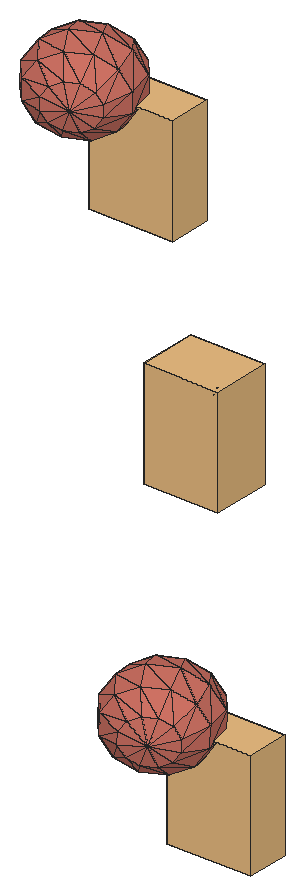
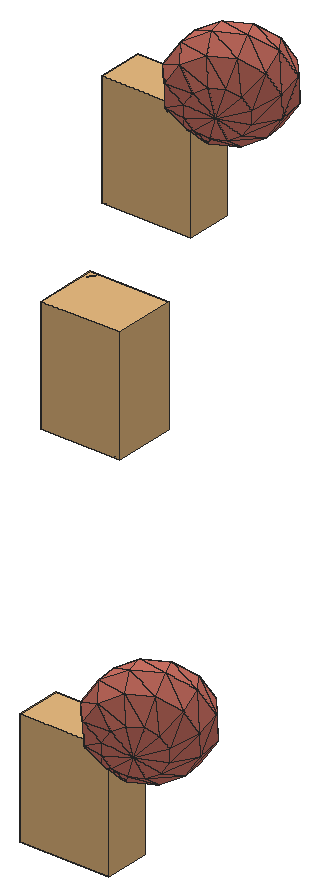
# SketchUp Ruby script. Lengths in inches.
U = 1.inch
M = Sketchup.active_model
def pt(a) = Geom::Point3d.new(a.map { |v| v * U })
def face(e, loops, mat)
  f = e.add_face(loops[0].map { |a| pt(a) })
  loops[1..].each { |l| e.add_face(l.map { |a| pt(a) }).erase! }
  f.material = f.back_material = mat if mat
  f
end
# faces: each face lists its corners as indices into pts; further lists are holes
def faces(e, pts, list, mat = nil) = list.each { |f| face(e, (f[0].is_a?(Array) ? f : [f]).map { |l| l.map { |i| pts[i] } }, mat) }
# xy, xz, yz: faces in a plane at the given z, y or x. An outline is a flat list of corners, or four numbers for a rectangle; further outlines are holes
def ring(l) = l.size == 4 ? [[l[0], l[1]], [l[2], l[1]], [l[2], l[3]], [l[0], l[3]]] : l.each_slice(2).to_a
def flat(e, list, mat, &to3) = list.each { |f| face(e, (f[0].is_a?(Array) ? f : [f]).map { |l| ring(l).map { |u, v| to3.(u, v) } }, mat) }
def xy(e, z, list, mat = nil) = flat(e, list, mat) { |x, y| [x, y, z] }
def xz(e, y, list, mat = nil) = flat(e, list, mat) { |x, z| [x, y, z] }
def yz(e, x, list, mat = nil) = flat(e, list, mat) { |y, z| [x, y, z] }
def lines(e, pts, list) = list.each { |a, b| e.add_line(pt(pts[a]), pt(pts[b])) }
# prism: a flat outline (further loops are holes) pulled along v
def prism(e, loops, v, mat = nil)
  f = face(e, loops, mat); d = Geom::Vector3d.new(v.map { |x| x * U })
  f.pushpull(f.normal.samedirection?(d) ? d.length : -d.length)
end
def box(e, o, s, mat = nil) = prism(e, [[o, [o[0] + s[0], o[1], o[2]], [o[0] + s[0], o[1] + s[1], o[2]], [o[0], o[1] + s[1], o[2]]]], [0, 0, s[2]], mat)
def at(x, y, z, deg = 0) = Geom::Transformation.translation(pt([x, y, z])) * Geom::Transformation.rotation(ORIGIN, Z_AXIS, deg.degrees)
def axes(o, x, y, z) = Geom::Transformation.new([*x, 0, *y, 0, *z, 0, *pt(o).to_a, 1])
def part(name) = M.definitions.add(name)
# library, detail: a bought-in or finely detailed component or shape, given as its bounding box
def library(name, o, s) = part(name).tap { |d| box(d.entities, o, s) }
def detail(e, o, s) = box(e.add_group.entities, o, s)
def put(e, d, t, mat = nil) = e.add_instance(d, t).tap { |i| i.material = mat if mat }
def group(e, t, mat = nil) = e.add_group.tap { |g| g.transformation = t; g.material = mat if mat }.entities
root = M.entities
M.materials.add("green").color = [174, 139, 102]
M.materials.add("vio").color = [206, 114, 100]
c1 = part("3DGeom~219_Defintion")
p = [[167.16,-297.35,-320.32],[-80.93,-262.73,-388.47],[-36.76,-95.49,-489.125],[218.17,-104.25,-436.54],[-281.83,-61.15,-410.64],[-43.21,95.93,-488.48],
  [-285.56,49.37,-410.27],[210.71,116.79,-435.8],[-317.52,144.24,-351.51],[-98.5625,260.26,-386.7],[-98.5625,260.26,-386.7],[370.46,-252.3,-166.34],
  [370.46,-252.3,-166.34],[414.63,-85.07,-266.99],[414.63,-85.07,-266.99],[414.63,-85.07,-266.99],[408.18,106.36,-266.34],[408.18,106.36,-266.34],
  [146.8,306.54,-318.28],[-98.5625,260.26,-386.7],[146.8,306.54,-318.28],[-307.34,-157.7,-352.53],[-281.83,-61.15,-410.64],[-307.34,-157.7,-352.53],
  [-451.39,-10.42,-222.13],[-285.56,49.37,-410.27],[-281.83,-61.15,-410.64],[-317.52,144.24,-351.51],[-285.56,49.37,-410.27],[71.36,-410.78,-118.27],
  [-163.89,-360.96,-213.49],[-80.93,-262.73,-388.47],[-80.93,-262.73,-388.47],[167.16,-297.35,-320.32],[-163.89,-360.96,-213.49],[-98.5625,260.26,-386.7],
  [-369.14,198.04,-250.11],[-98.5625,260.26,-386.7],[-369.14,198.04,-250.11],[-187.98,353.45,-211.07],[146.8,306.54,-318.28],[-98.5625,260.26,-386.7],
  [-187.98,353.45,-211.07],[-163.89,-360.96,-213.49],[-355.23,-214.42,-251.51],[-307.34,-157.7,-352.53],[-355.23,-214.42,-251.51],[-369.14,198.04,-250.11],
  [-317.52,144.24,-351.51],[287.5,-350.53,8.64],[167.16,-297.35,-320.32],[287.5,-350.53,8.64],[167.16,-297.35,-320.32],[370.46,-252.3,-166.34],
  [408.18,106.36,-266.34],[146.8,306.54,-318.28],[352.83,270.68,-164.57],[352.83,270.68,-164.57],[43.55,414.14,-115.47],[474.5,-139.65,32.21],
  [370.46,-252.3,-166.34],[414.63,-85.07,-266.99],[500,-43.09,-25.9],[408.18,106.36,-266.34],[496.27,67.43,-25.53],[352.83,270.68,-164.57],
  [-263.41,-363.87,-11.0625],[-412.69,-216.1,-134.63],[-355.23,-214.42,-251.51],[-355.23,-214.42,-251.51],[-355.23,-214.42,-251.51],[-412.69,-216.1,-134.63],
  [-426.6,196.36,-133.24],[-187.98,353.45,-211.07],[-412.69,-216.1,-134.63],[-464.32,-162.3,-33.23],[-496.27,-67.42,25.53],[-500,43.09,25.9],
  [-474.5,139.65,-32.21],[-43.55,-414.14,115.47],[-187.98,353.45,-211.07],[-287.5,350.54,-8.64],[-287.5,350.54,-8.64],[426.6,-196.36,133.24],
  [287.5,-350.53,8.64],[464.32,162.3,33.23],[263.41,363.87,11.0625],[352.83,270.68,-164.57],[263.41,363.87,11.0625],[-352.83,-270.68,164.57],
  [-412.69,-216.1,-134.63],[-263.41,-363.87,-11.0625],[-352.83,-270.68,164.57],[-412.69,-216.1,-134.63],[-287.5,350.54,-8.64],[187.98,-353.45,211.07],
  [187.98,-353.45,211.07],[287.5,-350.53,8.64],[-71.36,410.78,118.27],[-408.18,-106.36,266.34],[-352.83,-270.68,164.57],[-408.18,-106.36,266.34],
  [-370.46,252.3,166.34],[-287.5,350.54,-8.64],[-370.46,252.3,166.34],[451.39,10.42,222.13],[-146.8,-306.54,318.28],[-146.8,-306.54,318.28],
  [-352.83,-270.68,164.57],[-370.46,252.3,166.34],[369.14,-198.04,250.11],[187.98,-353.45,211.07],[263.41,363.87,11.0625],[412.69,216.1,134.63],
  [412.69,216.1,134.63],[163.89,360.96,213.49],[163.89,360.96,213.49],[-414.63,85.07,266.99],[-408.18,-106.36,266.34],[-414.63,85.07,266.99],
  [-370.46,252.3,166.34],[-414.63,85.07,266.99],[98.5625,-260.26,386.7],[-146.8,-306.54,318.28],[98.5625,-260.26,386.7],[187.98,-353.45,211.07],
  [-370.46,252.3,166.34],[-167.16,297.35,320.32],[163.89,360.96,213.49],[-167.16,297.35,320.32],[355.23,214.42,251.51],[412.69,216.1,134.63],
  [163.89,360.96,213.49],[355.23,214.42,251.51],[-210.71,-116.79,435.8],[-352.83,-270.68,164.57],[-146.8,-306.54,318.28],[-408.18,-106.36,266.34],
  [-167.16,297.35,320.32],[-370.46,252.3,166.34],[-414.63,85.07,266.99],[317.52,-144.24,351.51],[98.5625,-260.26,386.7],[187.98,-353.45,211.07],
  [317.52,-144.24,351.51],[187.98,-353.45,211.07],[369.14,-198.04,250.11],[355.23,214.42,251.51],[163.89,360.96,213.49],[80.93,262.73,388.47],
  [163.89,360.96,213.49],[-167.16,297.35,320.32],[80.93,262.73,388.47],[317.52,-144.24,351.51],[285.56,-49.37,410.27],[281.83,61.15,410.64],
  [307.34,157.7,352.53],[355.23,214.42,251.51],[307.34,157.7,352.53],[-218.17,104.25,436.54],[43.21,-95.93,488.48],[285.56,-49.37,410.27],
  [317.52,-144.24,351.51],[307.34,157.7,352.53],[36.76,95.49,489.125],[281.83,61.15,410.64],[307.34,157.7,352.53],[285.56,-49.37,410.27],
  [281.83,61.15,410.64],[285.56,-49.37,410.27],[281.83,61.15,410.64]]
faces(c1.entities,p,[[0,1,2],[0,2,3],[1,4,2],[3,2,5],[2,4,6],[2,6,5],[3,5,7],[5,6,8],
  [5,8,9],[7,5,10],[11,0,3],[12,3,13],[14,3,7],[15,7,16],[17,7,18],[7,19,20],
  [1,21,4],[22,23,24],[25,26,24],[27,28,24],[29,30,31],[29,32,33],[34,21,1],[35,8,36],
  [37,38,39],[40,41,42],[43,44,21],[45,46,24],[47,48,24],[49,29,50],[51,52,53],[54,55,56],
  [57,40,58],[40,42,58],[59,60,61],[59,61,62],[62,61,63],[62,63,64],[64,63,65],[66,67,68],
  [66,69,30],[70,71,24],[72,47,24],[73,47,72],[74,75,24],[75,76,24],[76,77,24],[77,78,24],
  [78,72,24],[79,66,30],[79,30,29],[80,72,81],[58,42,82],[83,84,60],[83,60,59],[64,65,85],
  [85,65,86],[87,58,88],[89,90,91],[92,75,93],[94,72,78],[95,79,29],[96,29,97],[58,82,98],
  [88,58,98],[99,75,100],[101,76,75],[102,78,77],[103,78,104],[59,62,105],[62,64,105],[64,85,105],
  [106,66,79],[107,108,66],[98,82,109],[110,111,84],[110,84,83],[85,112,113],[114,88,115],[88,98,116],
  [117,76,118],[119,77,76],[120,77,121],[83,59,105],[85,113,105],[122,123,79],[124,79,125],[98,126,127],
  [128,98,129],[110,83,105],[113,130,105],[131,132,133],[134,135,136],[134,137,135],[138,139,140],[141,142,143],
  [144,145,146],[147,148,149],[150,151,152],[153,110,105],[154,153,105],[155,154,105],[156,155,105],[130,156,105],
  [157,149,158],[159,137,134],[159,140,137],[138,140,159],[160,134,136],[160,136,142],[149,138,159],[161,142,162],
  [163,164,165],[166,149,164],[167,160,142],[149,159,164],[168,160,169],[170,164,160],[164,159,134],[164,134,160]],"vio")
c2 = library("3DGeom~96_Defintion",[-195.05,-500,-388.01],[390.1,1000,776.02])
c3 = part("3DGeom~97_Defintion")
p = [[174.48,487.39,-384.2],[155.8125,487.85,-388.01],[137.83,489.88,-382.14],[174.48,487.39,-384.2],[125.36,492.93,-368.18],[121.74,496.1875,-349.85],
  [174.48,487.39,-384.2],[121.74,496.1875,-349.85],[127.94,498.77,-332.09],[174.48,487.39,-384.2],[137.83,489.88,-382.14],[125.36,492.93,-368.18],
  [174.48,487.39,-384.2],[127.94,498.77,-332.09],[142.3,500,-319.63],[174.48,487.39,-384.2],[142.3,500,-319.63],[160.98,499.54,-315.83],
  [174.48,487.39,-384.2],[160.98,499.54,-315.83],[178.96,497.51,-321.7],[174.48,487.39,-384.2],[191.43,494.46,-335.66],[195.05,491.2,-353.98],
  [174.48,487.39,-384.2],[195.05,491.2,-353.98],[188.85,488.61,-371.75],[174.48,487.39,-384.2],[178.96,497.51,-321.7],[191.43,494.46,-335.66],
  [-147.29,-500,333.96],[-182.28,-490.37,332.19],[-165.51,-497.625,329.13],[-182.28,-490.37,332.19],[-147.29,-500,333.96],[-195.05,-469.79,356.79],
  [-182.28,-490.37,332.19],[-195.05,-469.79,356.79],[-193.09,-480.18,342.3125],[-195.05,-469.79,356.79],[-147.29,-500,333.96],[-172.82,-458.84,383.18],
  [-172.82,-458.84,383.18],[-147.29,-500,333.96],[-137.83,-468.47,384.95],[-147.29,-500,333.96],[-132.48,-496.86,345.39],[-125.0625,-489.05,360.34],
  [-137.83,-468.47,384.95],[-147.29,-500,333.96],[-125.0625,-489.05,360.34],[-195.05,-469.79,356.79],[-172.82,-458.84,383.18],[-187.63,-461.98,371.75],
  [-137.83,-468.47,384.95],[-125.0625,-489.05,360.34],[-127.02,-478.66,374.83],[-172.82,-458.84,383.18],[-137.83,-468.47,384.95],[-154.59,-461.21,388.01]]
faces(c3.entities,p,[[0,1,2],[3,4,5],[6,7,8],[9,10,11],[12,13,14],[15,16,17],[18,19,20],[21,22,23],
  [24,25,26],[27,28,29],[30,31,32],[33,34,35],[36,37,38],[39,40,41],[42,43,44],[45,46,47],
  [48,49,50],[51,52,53],[54,55,56],[57,58,59]],"green")
c4 = part("3DGeom~218_Defintion")
p = [[167.16,-297.35,-320.32],[-80.93,-262.73,-388.47],[-36.76,-95.49,-489.125],[218.17,-104.25,-436.54],[-281.83,-61.15,-410.64],[-43.21,95.93,-488.48],
  [-285.56,49.37,-410.27],[210.71,116.79,-435.8],[-317.52,144.24,-351.51],[-98.5625,260.26,-386.7],[-98.5625,260.26,-386.7],[370.46,-252.3,-166.34],
  [370.46,-252.3,-166.34],[414.63,-85.07,-266.99],[414.63,-85.07,-266.99],[414.63,-85.07,-266.99],[408.18,106.36,-266.34],[408.18,106.36,-266.34],
  [146.8,306.54,-318.28],[-98.5625,260.26,-386.7],[146.8,306.54,-318.28],[-307.34,-157.7,-352.53],[-281.83,-61.15,-410.64],[-307.34,-157.7,-352.53],
  [-451.39,-10.42,-222.13],[-285.56,49.37,-410.27],[-281.83,-61.15,-410.64],[-317.52,144.24,-351.51],[-285.56,49.37,-410.27],[71.36,-410.78,-118.27],
  [-163.89,-360.96,-213.49],[-80.93,-262.73,-388.47],[-80.93,-262.73,-388.47],[167.16,-297.35,-320.32],[-163.89,-360.96,-213.49],[-98.5625,260.26,-386.7],
  [-369.14,198.04,-250.11],[-98.5625,260.26,-386.7],[-369.14,198.04,-250.11],[-187.98,353.45,-211.07],[146.8,306.54,-318.28],[-98.5625,260.26,-386.7],
  [-187.98,353.45,-211.07],[-163.89,-360.96,-213.49],[-355.23,-214.42,-251.51],[-307.34,-157.7,-352.53],[-355.23,-214.42,-251.51],[-369.14,198.04,-250.11],
  [-317.52,144.24,-351.51],[287.5,-350.53,8.64],[167.16,-297.35,-320.32],[287.5,-350.53,8.64],[167.16,-297.35,-320.32],[370.46,-252.3,-166.34],
  [408.18,106.36,-266.34],[146.8,306.54,-318.28],[352.83,270.68,-164.57],[352.83,270.68,-164.57],[43.55,414.14,-115.47],[474.5,-139.65,32.21],
  [370.46,-252.3,-166.34],[414.63,-85.07,-266.99],[500,-43.09,-25.9],[408.18,106.36,-266.34],[496.27,67.43,-25.53],[352.83,270.68,-164.57],
  [-263.41,-363.87,-11.0625],[-412.69,-216.1,-134.63],[-355.23,-214.42,-251.51],[-355.23,-214.42,-251.51],[-355.23,-214.42,-251.51],[-412.69,-216.1,-134.63],
  [-426.6,196.36,-133.24],[-187.98,353.45,-211.07],[-412.69,-216.1,-134.63],[-464.32,-162.3,-33.23],[-496.27,-67.42,25.53],[-500,43.09,25.9],
  [-474.5,139.65,-32.21],[-43.55,-414.14,115.47],[-187.98,353.45,-211.07],[-287.5,350.54,-8.64],[-287.5,350.54,-8.64],[426.6,-196.36,133.24],
  [287.5,-350.53,8.64],[464.32,162.3,33.23],[263.41,363.87,11.0625],[352.83,270.68,-164.57],[263.41,363.87,11.0625],[-352.83,-270.68,164.57],
  [-412.69,-216.1,-134.63],[-263.41,-363.87,-11.0625],[-352.83,-270.68,164.57],[-412.69,-216.1,-134.63],[-287.5,350.54,-8.64],[187.98,-353.45,211.07],
  [187.98,-353.45,211.07],[287.5,-350.53,8.64],[-71.36,410.78,118.27],[-408.18,-106.36,266.34],[-352.83,-270.68,164.57],[-408.18,-106.36,266.34],
  [-370.46,252.3,166.34],[-287.5,350.54,-8.64],[-370.46,252.3,166.34],[451.39,10.42,222.13],[-146.8,-306.54,318.28],[-146.8,-306.54,318.28],
  [-352.83,-270.68,164.57],[-370.46,252.3,166.34],[369.14,-198.04,250.11],[187.98,-353.45,211.07],[263.41,363.87,11.0625],[412.69,216.1,134.63],
  [412.69,216.1,134.63],[163.89,360.96,213.49],[163.89,360.96,213.49],[-414.63,85.07,266.99],[-408.18,-106.36,266.34],[-414.63,85.07,266.99],
  [-370.46,252.3,166.34],[-414.63,85.07,266.99],[98.5625,-260.26,386.7],[-146.8,-306.54,318.28],[98.5625,-260.26,386.7],[187.98,-353.45,211.07],
  [-370.46,252.3,166.34],[-167.16,297.35,320.32],[163.89,360.96,213.49],[-167.16,297.35,320.32],[355.23,214.42,251.51],[412.69,216.1,134.63],
  [163.89,360.96,213.49],[355.23,214.42,251.51],[-210.71,-116.79,435.8],[-352.83,-270.68,164.57],[-146.8,-306.54,318.28],[-408.18,-106.36,266.34],
  [-167.16,297.35,320.32],[-370.46,252.3,166.34],[-414.63,85.07,266.99],[317.52,-144.24,351.51],[98.5625,-260.26,386.7],[187.98,-353.45,211.07],
  [317.52,-144.24,351.51],[187.98,-353.45,211.07],[369.14,-198.04,250.11],[355.23,214.42,251.51],[163.89,360.96,213.49],[80.93,262.73,388.47],
  [163.89,360.96,213.49],[-167.16,297.35,320.32],[80.93,262.73,388.47],[317.52,-144.24,351.51],[285.56,-49.37,410.27],[281.83,61.15,410.64],
  [307.34,157.7,352.53],[355.23,214.42,251.51],[307.34,157.7,352.53],[-218.17,104.25,436.54],[43.21,-95.93,488.48],[285.56,-49.37,410.27],
  [317.52,-144.24,351.51],[307.34,157.7,352.53],[36.76,95.49,489.125],[281.83,61.15,410.64],[307.34,157.7,352.53],[285.56,-49.37,410.27],
  [281.83,61.15,410.64],[285.56,-49.37,410.27],[281.83,61.15,410.64]]
faces(c4.entities,p,[[0,1,2],[0,2,3],[1,4,2],[3,2,5],[2,4,6],[2,6,5],[3,5,7],[5,6,8],
  [5,8,9],[7,5,10],[11,0,3],[12,3,13],[14,3,7],[15,7,16],[17,7,18],[7,19,20],
  [1,21,4],[22,23,24],[25,26,24],[27,28,24],[29,30,31],[29,32,33],[34,21,1],[35,8,36],
  [37,38,39],[40,41,42],[43,44,21],[45,46,24],[47,48,24],[49,29,50],[51,52,53],[54,55,56],
  [57,40,58],[40,42,58],[59,60,61],[59,61,62],[62,61,63],[62,63,64],[64,63,65],[66,67,68],
  [66,69,30],[70,71,24],[72,47,24],[73,47,72],[74,75,24],[75,76,24],[76,77,24],[77,78,24],
  [78,72,24],[79,66,30],[79,30,29],[80,72,81],[58,42,82],[83,84,60],[83,60,59],[64,65,85],
  [85,65,86],[87,58,88],[89,90,91],[92,75,93],[94,72,78],[95,79,29],[96,29,97],[58,82,98],
  [88,58,98],[99,75,100],[101,76,75],[102,78,77],[103,78,104],[59,62,105],[62,64,105],[64,85,105],
  [106,66,79],[107,108,66],[98,82,109],[110,111,84],[110,84,83],[85,112,113],[114,88,115],[88,98,116],
  [117,76,118],[119,77,76],[120,77,121],[83,59,105],[85,113,105],[122,123,79],[124,79,125],[98,126,127],
  [128,98,129],[110,83,105],[113,130,105],[131,132,133],[134,135,136],[134,137,135],[138,139,140],[141,142,143],
  [144,145,146],[147,148,149],[150,151,152],[153,110,105],[154,153,105],[155,154,105],[156,155,105],[130,156,105],
  [157,149,158],[159,137,134],[159,140,137],[138,140,159],[160,134,136],[160,136,142],[149,138,159],[161,142,162],
  [163,164,165],[166,149,164],[167,160,142],[149,159,164],[168,160,169],[170,164,160],[164,159,134],[164,134,160]],"vio")
c5 = library("3DGeom~94_Defintion",[-195.05,-500,-388.01],[390.1,1000,776.02])
c6 = part("3DGeom~95_Defintion")
p = [[174.48,487.39,-384.2],[155.8125,487.85,-388.01],[137.83,489.88,-382.14],[174.48,487.39,-384.2],[125.36,492.93,-368.18],[121.74,496.1875,-349.85],
  [174.48,487.39,-384.2],[121.74,496.1875,-349.85],[127.94,498.77,-332.09],[174.48,487.39,-384.2],[137.83,489.88,-382.14],[125.36,492.93,-368.18],
  [174.48,487.39,-384.2],[127.94,498.77,-332.09],[142.3,500,-319.63],[174.48,487.39,-384.2],[142.3,500,-319.63],[160.98,499.54,-315.83],
  [174.48,487.39,-384.2],[160.98,499.54,-315.83],[178.96,497.51,-321.7],[174.48,487.39,-384.2],[191.43,494.46,-335.66],[195.05,491.2,-353.98],
  [174.48,487.39,-384.2],[195.05,491.2,-353.98],[188.85,488.61,-371.75],[174.48,487.39,-384.2],[178.96,497.51,-321.7],[191.43,494.46,-335.66],
  [-147.28,-500,333.96],[-182.28,-490.37,332.19],[-165.51,-497.625,329.13],[-182.28,-490.37,332.19],[-147.28,-500,333.96],[-195.05,-469.79,356.79],
  [-182.28,-490.37,332.19],[-195.05,-469.79,356.79],[-193.09,-480.18,342.3125],[-195.05,-469.79,356.79],[-147.28,-500,333.96],[-172.82,-458.84,383.18],
  [-172.82,-458.84,383.18],[-147.28,-500,333.96],[-137.83,-468.47,384.95],[-147.28,-500,333.96],[-132.48,-496.86,345.39],[-125.06,-489.05,360.34],
  [-137.83,-468.47,384.95],[-147.28,-500,333.96],[-125.06,-489.05,360.34],[-195.05,-469.79,356.79],[-172.82,-458.84,383.18],[-187.63,-461.98,371.75],
  [-137.83,-468.47,384.95],[-125.06,-489.05,360.34],[-127.02,-478.66,374.83],[-172.82,-458.84,383.18],[-137.83,-468.47,384.95],[-154.59,-461.21,388.01]]
faces(c6.entities,p,[[0,1,2],[3,4,5],[6,7,8],[9,10,11],[12,13,14],[15,16,17],[18,19,20],[21,22,23],
  [24,25,26],[27,28,29],[30,31,32],[33,34,35],[36,37,38],[39,40,41],[42,43,44],[45,46,47],
  [48,49,50],[51,52,53],[54,55,56],[57,58,59]],"green")
c7 = library("3DGeom~74_Defintion",[-269.59,-500,-344.14],[539.17,1000,688.28])
c8 = part("3DGeom~75_Defintion")
p = [[-217.33,-469.79,-343.43],[-251.16,-458.84,-336.67],[-234.01,-461.98,-344.14],[-217.33,-469.79,-343.43],[-220.35,-500,-290.57],[-251.16,-458.84,-336.67],
  [-201.93,-490.37,-320.375],[-201.93,-490.37,-320.375],[-217.33,-469.79,-343.43],[-205.59,-480.18,-334.73],[-269.59,-468.47,-306.87],[-251.16,-458.84,-336.67],
  [-269.59,-468.47,-306.87],[-264.18,-461.21,-323.03],[-220.35,-500,-290.57],[-201.93,-490.37,-320.375],[-207.33,-497.625,-304.21],[-254.18,-489.05,-283.82],
  [-269.59,-468.47,-306.87],[-254.18,-489.05,-283.82],[-265.93,-478.66,-292.52],[-220.35,-500,-290.57],[-237.5,-496.86,-283.11],[-254.18,-489.05,-283.82],
  [253.72,487.39,337.56],[230.5,498.77,271.66],[212.66,500,278.24],[253.72,487.39,337.56],[249.06,496.1875,274.79],[230.5,498.77,271.66],
  [253.72,487.39,337.56],[263.36,492.93,286.79],[249.06,496.1875,274.79],[253.72,487.39,337.56],[212.66,500,278.24],[200.33,499.54,292.76],
  [253.72,487.39,337.56],[269.58,489.88,304.45],[263.36,492.93,286.79],[253.72,487.39,337.56],[200.33,499.54,292.76],[196.8,497.51,311.34],
  [253.72,487.39,337.56],[266.06,487.85,323.03],[269.58,489.88,304.45],[253.72,487.39,337.56],[196.8,497.51,311.34],[203.02,494.46,329],
  [253.72,487.39,337.56],[203.02,494.46,329],[217.33,491.2,341.01],[253.72,487.39,337.56],[217.33,491.2,341.01],[235.89,488.61,344.14]]
faces(c8.entities,p,[[0,1,2],[3,4,5],[6,4,3],[7,8,9],[5,4,10],[11,12,13],[14,15,16],[10,4,17],
  [18,19,20],[21,22,23],[24,25,26],[27,28,29],[30,31,32],[33,34,35],[36,37,38],[39,40,41],
  [42,43,44],[45,46,47],[48,49,50],[51,52,53]],"green")
g1 = group(root,at(15.3125,38.42,26.21))
put(g1,c1,axes([-2.11,-0.4,15.58],[0,0.00039,0],[0,0,-0.00039],[-0.00039,0,0]),"vio")
g2 = group(root,at(15.3125,38.42,26.21))
put(g2,c2,axes([-1.94,-0.32,15.36],[0,0.0004,0],[0,0,-0.0004],[-0.0004,0,0]),"green")
put(g2,c3,axes([-1.94,-0.32,15.36],[0,0.0004,0],[0,0,-0.0004],[-0.0004,0,0]),"green")
g3 = group(root,at(15.3125,38.42,26.21))
put(g3,c4,axes([-1.88,-0.33,13.53],[0,0.00039,0],[0,0,-0.00039],[-0.00039,0,0]),"vio")
g4 = group(root,at(15.3125,38.42,26.21))
put(g4,c5,axes([-1.71,-0.25,13.31],[0,0.0004,0],[0,0,-0.0004],[-0.0004,0,0]),"green")
put(g4,c6,axes([-1.71,-0.25,13.31],[0,0.0004,0],[0,0,-0.0004],[-0.0004,0,0]),"green")
g5 = group(root,at(15.3125,38.42,26.21))
put(g5,c7,axes([-1.7,-0.36,14.57],[0,0.0004,0],[0,0,-0.0004],[-0.0004,0,0]),"green")
put(g5,c8,axes([-1.7,-0.36,14.57],[0,0.0004,0],[0,0,-0.0004],[-0.0004,0,0]),"green")
